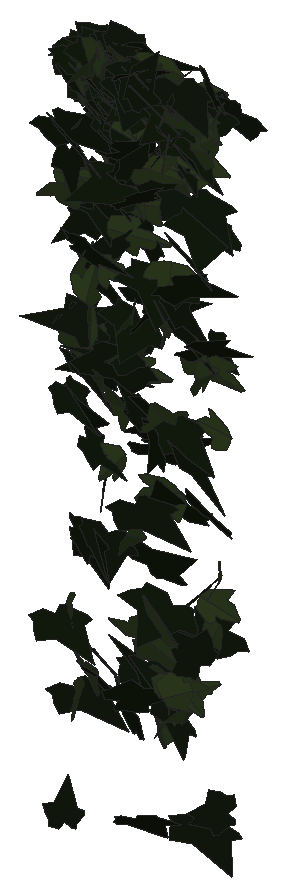
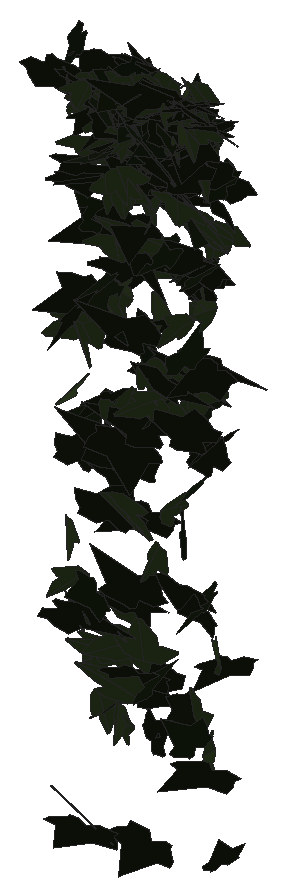
# SketchUp Ruby script. Lengths in millimetres.
U = 1.mm
M = Sketchup.active_model
def pt(a) = Geom::Point3d.new(a.map { |v| v * U })
def face(e, loops, mat)
  f = e.add_face(loops[0].map { |a| pt(a) })
  loops[1..].each { |l| e.add_face(l.map { |a| pt(a) }).erase! }
  f.material = f.back_material = mat if mat
  f
end
# faces: each face lists its corners as indices into pts; further lists are holes
def faces(e, pts, list, mat = nil) = list.each { |f| face(e, (f[0].is_a?(Array) ? f : [f]).map { |l| l.map { |i| pts[i] } }, mat) }
# xy, xz, yz: faces in a plane at the given z, y or x. An outline is a flat list of corners, or four numbers for a rectangle; further outlines are holes
def ring(l) = l.size == 4 ? [[l[0], l[1]], [l[2], l[1]], [l[2], l[3]], [l[0], l[3]]] : l.each_slice(2).to_a
def flat(e, list, mat, &to3) = list.each { |f| face(e, (f[0].is_a?(Array) ? f : [f]).map { |l| ring(l).map { |u, v| to3.(u, v) } }, mat) }
def xy(e, z, list, mat = nil) = flat(e, list, mat) { |x, y| [x, y, z] }
def xz(e, y, list, mat = nil) = flat(e, list, mat) { |x, z| [x, y, z] }
def yz(e, x, list, mat = nil) = flat(e, list, mat) { |y, z| [x, y, z] }
def lines(e, pts, list) = list.each { |a, b| e.add_line(pt(pts[a]), pt(pts[b])) }
# prism: a flat outline (further loops are holes) pulled along v
def prism(e, loops, v, mat = nil)
  f = face(e, loops, mat); d = Geom::Vector3d.new(v.map { |x| x * U })
  f.pushpull(f.normal.samedirection?(d) ? d.length : -d.length)
end
def box(e, o, s, mat = nil) = prism(e, [[o, [o[0] + s[0], o[1], o[2]], [o[0] + s[0], o[1] + s[1], o[2]], [o[0], o[1] + s[1], o[2]]]], [0, 0, s[2]], mat)
def at(x, y, z, deg = 0) = Geom::Transformation.translation(pt([x, y, z])) * Geom::Transformation.rotation(ORIGIN, Z_AXIS, deg.degrees)
def axes(o, x, y, z) = Geom::Transformation.new([*x, 0, *y, 0, *z, 0, *pt(o).to_a, 1])
def part(name) = M.definitions.add(name)
# library, detail: a bought-in or finely detailed component or shape, given as its bounding box
def library(name, o, s) = part(name).tap { |d| box(d.entities, o, s) }
def detail(e, o, s) = box(e.add_group.entities, o, s)
def put(e, d, t, mat = nil) = e.add_instance(d, t).tap { |i| i.material = mat if mat }
def group(e, t, mat = nil) = e.add_group.tap { |g| g.transformation = t; g.material = mat if mat }.entities
root = M.entities
M.materials.add("efeu1").color = [18, 25, 13]
M.materials.add("efeu2").color = [43, 57, 29]
c1 = part("ivyleaf_9")
p = [[39.1,54.8,31.7],[34.5,51.8,30.2],[-5.3,25.2,17.3],[-17.9,28.3,20.9],[-21.6,21.7,17],[-20.2,4.3,5.3],
  [-22.9,-0.3,2.5],[-17.1,-4,-0.6],[-2,-2.1,-1.2],[-0.7,-15.4,-10.1],[16.6,-22.3,-16.7],[21.1,-15.1,-12.5],
  [32.7,-10.7,-11],[46.1,-1.8,-6.6],[30.8,11.2,3.8]]
faces(c1.entities,p,[[0,1,2,3,4,5,6,7,8,9,10,11,12,13,14]],"efeu1")
c2 = part("ivyleaf_10")
p = [[0,12.8,-0.8],[-1.5,51.3,-10.9],[-4.9,51,-11.6],[-13.6,26.5,-7.3],[-13.2,15.9,-4.6],[-21.1,19.3,-7.2],
  [-29.5,16.3,-8.3],[-29.2,8.3,-6.2],[-19.7,-9.8,0.5],[-7.6,-13,4],[1,-12.2,5.8],[-0.4,51.1,-11.1],
  [-1.5,51.1,-10.9],[1,-12.4,5.9],[16.9,-12.4,3.5],[35.1,9.1,-5.1],[35,12.9,-6.1],[20.5,16.4,-4.9],
  [15.8,15,-3.8],[15.3,27.6,-7.1],[12.8,31.3,-7.8]]
faces(c2.entities,p,[[0,1,2,3,4,5,6,7,8,9,10],[11,12,0,13,14,15,16,17,18,19,20]],"efeu2")
put(root,c1,axes([3016.5,906.6,724.8],[0.03199,-0.66358,-0.6588],[-0.00347,0.65889,-0.66371],[1.77963,0.01322,0.01055]))
put(root,c1,axes([3235.8,920.3,1050.6],[0.77001,-0.91344,0.16816],[0.11583,-0.15696,-0.999],[1.76387,0.40906,-0.00781]))
put(root,c1,axes([3163.6,892,1496.8],[-0.15428,0.62413,0.77413],[-0.13659,0.771,-0.62913],[-1.88759,-0.1068,-0.01775]))
put(root,c1,axes([3119.7,925.8,1438],[-1.17393,-0.41882,0.51172],[-0.83195,-0.26683,-0.74529],[0.94432,-0.75573,-0.02045]))
put(root,c1,axes([3132.1,929.1,1585],[-0.45462,-0.7398,0.46488],[-0.03422,-0.47768,-0.76941],[1.66255,-0.21213,0.11129]))
put(root,c1,axes([3026,920.8,1459.1],[-0.74129,0.0016,-0.76927],[1.42556,-0.1957,-0.37966],[-0.33362,-0.83975,0.08701]))
put(root,c1,axes([3236.7,894.7,1333.6],[0.02355,0.26448,-0.88],[0.15228,0.87643,0.26454],[1.74218,-0.08018,-0.01122]))
put(root,c1,axes([3145.6,904.1,1598.4],[-1.12891,0.71334,0.38975],[0.45858,-0.30651,0.92768],[1.47753,0.64016,0.00987]))
put(root,c1,axes([3271.4,922.3,965.5],[1.1347,-0.65239,0.21976],[-0.27641,0.16498,0.88377],[-1.28069,-0.61363,0.00397]))
put(root,c2,axes([3021.4,927.9,733.6],[0.09927,-0.14231,-0.80456],[0.31208,-0.78798,0.15001],[-1.52338,-0.1707,-0.0217]))
put(root,c2,axes([3200,926.2,1527.2],[-0.00712,0.38664,-0.74683],[0.00939,-0.74681,-0.38666],[-1.60052,-0.0061,0.00105]))
put(root,c1,axes([3064.1,926,1574],[1.27825,-0.56394,-0.15563],[0.28866,-0.061,0.87557],[-1.07535,-0.68672,0.05003]))
put(root,c1,axes([3011.8,923.9,1489.2],[0.73758,-0.69043,0.3946],[0.33043,-0.35491,-0.79151],[1.47698,0.42419,-0.01998]))
put(root,c1,axes([3175.2,930.5,1048.2],[0.21099,-0.24209,-0.83674],[1.11722,-0.60241,0.25207],[-1.22479,-0.59121,0.08579]))
put(root,c1,axes([3136.7,900.5,635.8],[0.42934,0.04435,0.93346],[1.63406,0.3693,-0.22504],[-0.70222,0.88648,0.04705]))
put(root,c1,axes([3040.8,919.7,1317],[0.77704,-0.32089,0.63116],[0.90562,-0.41516,-0.51889],[0.99788,0.62665,-0.02057]))
put(root,c2,axes([3072.9,899,1260.7],[0.31768,0.55295,-0.67549],[0.18244,0.67195,0.57375],[1.65135,-0.18061,0.06656]))
put(root,c1,axes([3217.5,923,1554.7],[-0.80889,0.32031,-0.6481],[0.78398,-0.51052,-0.52245],[-1.13068,-0.58313,0.1014]))
put(root,c2,axes([3146.6,905.7,1250.1],[0.0201,-0.71991,-0.55145],[-0.0438,0.55109,-0.71989],[1.72535,0.02238,-0.01185]))
put(root,c2,axes([3065.2,924.6,1213.5],[0.01128,0.62166,-0.62218],[0.05319,-0.62201,-0.62123],[-1.67307,-0.01558,-0.02394]))
put(root,c1,axes([3223.8,929.5,1363.6],[0.26083,-0.60882,0.63453],[0.47113,-0.58951,-0.61909],[1.60594,0.27183,0.07857]))
put(root,c2,axes([3071.1,923.2,1107.6],[-1.08171,0.36184,0.57297],[0.83651,-0.37236,0.67114],[0.98166,0.71602,0.05947]))
put(root,c1,axes([3127.5,925,1160.2],[-0.02278,-0.04915,-0.96158],[-1.04023,-0.79135,0.04726],[-1.5086,0.5464,-0.01806]))
put(root,c1,axes([3140.7,932.1,1226.8],[-0.7383,-0.8102,0.2561],[-0.17966,-0.23869,-0.89811],[1.60715,-0.39888,0.01725]))
put(root,c1,axes([3028.2,908.9,404.5],[-0.60671,-0.39713,0.63358],[0.80336,0.47294,0.50883],[-1.17469,0.52856,0.02075]))
put(root,c1,axes([3167.3,925.1,1624.7],[-1.62137,-0.22979,-0.15515],[0.29372,0.02347,-0.88219],[0.43837,-0.86561,0.01726]))
put(root,c2,axes([3271.9,900.3,1197.8],[-0.09284,-0.21112,-0.88256],[0.39565,0.85773,-0.21667],[1.68115,-0.21352,0.00226]))
put(root,c1,axes([3147.5,899.8,1435.6],[0.79698,0.55323,0.53455],[0.59256,0.43467,-0.69376],[-1.33885,0.5217,0.01116]))
put(root,c2,axes([3026.5,914.1,1408.9],[-0.9948,-0.63536,-0.25479],[0.32696,0.18856,-0.82264],[1.26112,-0.55007,0.0123]))
put(root,c1,axes([3035.6,927.8,1127.1],[0.66585,-0.77664,0.20114],[0.21496,-0.16957,-0.85119],[1.51166,0.3662,0.03244]))
put(root,c2,axes([3207.5,912.1,756.8],[-1.03385,0.5754,-0.56238],[-0.75433,0.39914,0.79123],[1.33261,0.67234,0.01158]))
put(root,c2,axes([3065.5,913.8,1615.3],[-0.22834,-0.80416,-0.39552],[0.08826,0.39294,-0.81299],[1.70329,-0.12816,-0.01089]))
put(root,c1,axes([3150.3,932.7,1581.7],[0.31999,-0.57886,0.64341],[0.66315,-0.5547,-0.5901],[1.50779,0.36682,0.12299]))
put(root,c2,axes([3206.1,921.3,1334.5],[1.22811,0.5381,-0.09299],[-0.13681,-0.059,-0.84021],[-1.03024,0.64928,0.00072]))
put(root,c1,axes([3027.7,933.3,1048.1],[0.05351,-0.23036,0.88742],[0.72469,-0.80471,-0.22096],[1.58732,0.37516,0.07096]))
put(root,c1,axes([3066.6,926.1,1196.2],[-1.31861,0.12511,0.53559],[-1.01976,0.04091,-0.70268],[-0.23628,-0.87476,0.04374]))
put(root,c1,axes([3022.1,920.5,1082],[0.47438,-0.69712,-0.46598],[-0.30837,0.43693,-0.74033],[1.5658,0.29725,-0.00463]))
put(root,c2,axes([3211.4,921.6,682.1],[1.267,0.15294,0.54034],[0.97961,0.1689,-0.68197],[-0.42735,0.84061,0.03871]))
put(root,c2,axes([3219.8,909,671.3],[0.4764,0.20234,-0.90415],[1.31611,0.58252,0.32181],[1.17357,-0.73541,0.00614]))
put(root,c1,axes([3183.5,932.3,1309],[-1.2112,-0.66708,-0.29739],[0.39205,0.21449,-0.92196],[1.33361,-0.66891,0.00094]))
put(root,c2,axes([3034.2,924,1168.9],[-0.26087,-0.00409,-0.96092],[1.79905,-0.17506,-0.1341],[-0.32875,-0.95473,0.0287]))
put(root,c1,axes([3264.4,934.2,1420.5],[-1.06024,-0.68406,-0.15095],[0.19463,0.11137,-0.88216],[1.31895,-0.56632,0.00884]))
put(root,c2,axes([3121,913.8,1091.2],[0.69764,-0.22428,-0.77737],[-0.75589,0.69364,-0.38741],[1.34153,0.50747,0.18597]))
put(root,c1,axes([3208.9,933.6,1242.7],[0.79091,-0.76758,0.18436],[0.19312,-0.15468,-0.87272],[1.48995,0.42751,0.01525]))
put(root,c1,axes([3007.6,919.7,1504.4],[0.14455,-0.0471,-0.905],[1.13121,0.68814,0.01406],[1.30194,-0.59267,0.08826]))
put(root,c1,axes([3215.2,924,1086.1],[0.32906,-0.71736,-0.57502],[-0.18495,0.56756,-0.73727],[1.73995,0.196,0.03038]))
put(root,c1,axes([3086.7,935.3,1464.6],[-0.1513,-0.00027,0.88074],[0.91882,-0.73964,0.04335],[1.40196,0.48472,0.06664]))
put(root,c1,axes([3263.2,910.4,735.4],[-0.43663,0.59231,0.8468],[-0.6175,0.78226,-0.63507],[-1.86729,-0.39719,0.012]))
put(root,c1,axes([3215.3,928.6,1625.8],[-0.45933,-0.6222,-0.57073],[0.47956,0.51346,-0.66632],[1.53367,-0.3469,0.03741]))
put(root,c1,axes([3131.6,927.2,1177.7],[-1.51791,0.37027,0.39319],[-0.68532,0.15809,-0.87928],[-0.7661,-0.87505,0.00752]))
put(root,c1,axes([3151.1,926.6,1615.4],[1.34169,-0.49975,-0.12423],[-0.15909,0.09677,-0.8636],[0.96707,0.70926,0.03029]))
put(root,c2,axes([3050.7,934.9,628.1],[-1.03805,0.41996,0.55461],[0.84331,-0.33359,0.68835],[1.0207,0.70271,-0.00468]))
put(root,c1,axes([3127.2,914.3,1499.4],[1.12247,0.22043,0.72035],[1.26227,0.28189,-0.62928],[-0.67987,0.88729,0.02096]))
put(root,c2,axes([3158.4,919.7,1483.8],[-0.61294,-0.20641,-0.80724],[1.371,0.36593,-0.38097],[0.79688,-0.78832,0.03453]))
put(root,c1,axes([3205,927.3,1282.8],[0.90994,-0.6847,-0.38993],[-0.35624,0.34435,-0.83417],[1.4567,0.51192,0.03958]))
put(root,c2,axes([3023,945.8,591.7],[0.2596,-0.29183,0.87678],[0.80792,-0.76744,-0.32148],[1.56213,0.44541,0.02056]))
put(root,c1,axes([3205.2,943.4,1569.5],[-1.13814,-0.53068,0.26285],[-0.37501,-0.17398,-0.79953],[1.06289,-0.62964,-0.00062]))
put(root,c2,axes([3200.5,915,1251.7],[-0.17117,0.37181,-0.81824],[-0.568,0.76331,0.37965],[1.61345,0.30816,0.04685]))
put(root,c1,axes([3061.7,926.2,640.9],[1.49573,-0.2609,-0.21098],[-0.38053,0.06735,-0.82808],[0.51282,0.81094,0.0009]))
put(root,c1,axes([3250.1,916.2,1225.6],[1.06548,0.41629,0.59108],[0.91847,0.34146,-0.69757],[-1.02452,0.73905,-0.01065]))
put(root,c2,axes([3064.5,931.2,1627.5],[0.9873,-0.6228,-0.29877],[-0.37561,0.22443,-0.81051],[1.25984,0.55498,-0.00751]))
put(root,c1,axes([3187.5,931.6,1525.4],[-0.69255,0.6912,-0.30489],[0.27751,-0.26779,-0.78112],[-1.41075,-0.392,-0.00398]))
put(root,c1,axes([3142.9,929.8,1444.2],[-0.43917,-0.05903,0.8526],[1.59134,-0.19839,0.21256],[0.33667,0.86071,0.10747]))
put(root,c1,axes([3141.5,933.1,1077],[-0.23769,-0.72973,0.45929],[0.15503,0.45202,0.74033],[-1.63368,0.14907,0.00343]))
put(root,c1,axes([3189.4,947.2,613.8],[0.04591,-0.82645,0.28701],[0.05156,-0.28627,-0.82662],[1.66426,0.03167,0.01769]))
put(root,c1,axes([3185.7,944.3,783.6],[-1.56836,-0.48288,-0.08674],[0.13995,0.04608,-0.95511],[0.92317,-0.82733,-0.00257]))
put(root,c1,axes([3011.6,937.9,1573.3],[0.95627,-0.71675,-0.00209],[-0.00388,0.00112,-0.87532],[1.36411,0.50246,-0.00103]))
put(root,c2,axes([3011.1,934.6,1415.8],[0.26015,-0.19673,-0.77637],[1.4909,-0.1311,0.17114],[-0.31729,-0.77733,0.16762]))
put(root,c2,axes([3179.9,944.8,1071.6],[-0.80618,-0.63347,-0.44419],[-0.47773,-0.36649,0.76203],[-1.39283,0.49236,-0.00427]))
put(root,c1,axes([3181.4,946.8,1537.5],[0.55395,-0.77376,0.38072],[0.34464,-0.33802,-0.82542],[1.60464,0.33972,0.04585]))
put(root,c2,axes([3018.9,943.7,1573.3],[-0.79019,0.41173,-0.57655],[0.35845,-0.58007,-0.54987],[-1.29984,-0.41026,0.19885]))
put(root,c1,axes([3232,936.5,1449.2],[-0.55972,-0.5166,-0.75993],[0.94227,0.5831,-0.58799],[1.47329,-0.5692,0.08735]))
put(root,c2,axes([3225.2,931.8,1579],[-1.21506,-0.18733,-0.51249],[0.95175,0.11471,-0.6649],[0.41548,-0.8106,0.02435]))
put(root,c1,axes([3041.4,951.2,1353.8],[-0.05125,-0.00723,-0.85682],[0.44788,-0.82434,-0.00044],[-1.56805,-0.23522,0.02788]))
put(root,c2,axes([3042.8,919.1,1280.9],[0.31995,-0.30744,0.92992],[-0.61966,0.87232,0.34726],[-1.75802,-0.36342,0.04684]))
put(root,c2,axes([3122.1,949.8,1420.8],[-0.45389,0.26662,-0.79049],[0.49251,-0.75796,-0.33372],[-1.50942,-0.32749,0.12882]))
put(root,c2,axes([3182.1,936.2,1583.4],[0.68526,-0.77432,-0.22314],[-0.09085,0.22348,-0.85251],[1.53096,0.35985,0.04929]))
put(root,c2,axes([3255.5,953.6,1549],[-0.56066,0.2219,0.81755],[0.58302,-0.7791,0.32184],[1.50316,0.38495,0.18011]))
put(root,c1,axes([3139,932.5,930.1],[-0.16542,-0.34994,-0.84075],[0.67082,0.76582,-0.35519],[1.5981,-0.35768,0.06207]))
put(root,c2,axes([3170.5,936.2,716.6],[-1.50778,0.07311,-0.67145],[1.27343,-0.05628,-0.79559],[-0.17541,-1.03697,-0.00415]))
put(root,c1,axes([3129.9,926.5,1471.8],[-0.47597,0.51858,0.59693],[-0.51849,0.53123,-0.57564],[-1.41277,-0.36968,0.01015]))
put(root,c1,axes([3122.1,940.4,1606.2],[1.27898,-0.53776,0.07978],[0.11368,-0.05305,-0.86068],[1.0284,0.67466,-0.00408]))
put(root,c1,axes([3137.3,924.9,1619.8],[0.81769,0.74315,0.1304],[0.12793,0.11176,-0.8584],[-1.43026,0.43486,-0.00223]))
put(root,c1,axes([3050.4,934.4,1004.2],[0.85875,-0.53112,-0.52878],[-0.47761,0.47452,-0.69075],[1.34403,0.50797,0.09239]))
put(root,c1,axes([3217.1,941.5,1544.6],[-0.09698,-0.76734,-0.48789],[0.0211,0.48809,-0.76882],[1.73046,-0.04895,-0.01797]))
put(root,c2,axes([3185.1,952,1242.9],[0.58246,-0.68053,0.47277],[0.35148,-0.4353,-0.74613],[1.5374,0.35734,-0.00854]))
put(root,c1,axes([3106.4,939.8,1341.5],[-1.1618,0.56333,-0.07607],[0.10691,-0.05129,-0.83065],[-1.07656,-0.61303,-0.0004]))
put(root,c1,axes([3102.8,933.3,1578],[1.463,0.05488,-0.39208],[-0.75086,0.03492,-0.76862],[-0.06271,0.86221,0.05609]))
put(root,c1,axes([3055.5,953.4,1612.6],[-0.62933,-0.77131,0.05423],[-0.02561,-0.05323,-0.83916],[1.47135,-0.33083,0.00859]))
put(root,c1,axes([3129.6,935.5,576],[0.25378,-0.42054,0.73686],[-0.14931,0.7366,0.43459],[-1.6078,-0.13478,0.07595]))
put(root,c2,axes([3058.2,935.3,1601],[0.40126,-0.7276,-0.46431],[-0.00543,0.47738,-0.74936],[1.6427,0.17931,0.11094]))
put(root,c2,axes([3246.9,936.1,1532.1],[-0.60007,0.12301,0.8302],[-1.55694,0.15303,-0.33336],[-0.35675,-0.87477,0.05842]))
put(root,c1,axes([3258.2,935.3,1646.8],[0.99038,-0.38329,-0.62649],[-1.00202,0.34064,-0.64572],[0.97455,0.73976,-0.02726]))
put(root,c2,axes([3125.8,944.5,1166.8],[-0.42596,-0.92534,0.01728],[-0.00071,-0.01769,-0.95202],[1.76142,-0.22378,0.0038]))
put(root,c2,axes([3102.2,939.6,1626.1],[-1.31272,0.46227,-0.04073],[0.06058,-0.02565,-0.83032],[-0.88112,-0.69047,0.00358]))
put(root,c2,axes([3187.2,933.1,580.3],[0.71042,-0.29831,0.723],[-1.10589,0.43047,0.47761],[-0.99637,-0.69048,-0.0146]))
put(root,c2,axes([3249.5,939,1195.4],[-1.2336,-0.09948,-0.60288],[1.13359,0.09329,-0.65576],[0.25954,-0.88028,-0.00137]))
put(root,c1,axes([3094.9,947.7,1522.3],[-0.92806,-0.47094,-0.5863],[0.88455,0.36061,-0.67621],[1.12517,-0.67193,0.04801]))
put(root,c2,axes([3060.2,935,1421.9],[0.4104,-0.19118,-0.90246],[-1.32683,0.57316,-0.288],[1.14976,0.72967,-0.01023]))
put(root,c2,axes([3040.7,945.6,1514.4],[0.1265,-0.85038,-0.03459],[0.00369,0.03485,-0.85296],[1.61978,0.06633,0.00464]))
put(root,c1,axes([3099.8,961.4,1520.8],[-0.56583,-0.57673,0.50695],[-0.12178,-0.52312,-0.63265],[1.45631,-0.26783,0.14406]))
put(root,c1,axes([3148.1,945.6,676.5],[-0.48286,-0.54509,-0.63173],[0.61071,0.54577,-0.59979],[1.46589,-0.40693,0.04179]))
put(root,c2,axes([3135.9,948.2,717.8],[-1.62994,-0.13948,0.0913],[0.17289,0.01019,0.86769],[-0.26602,0.86121,0.00452]))
put(root,c2,axes([3278.6,935,862.5],[0.11288,-0.60517,-0.65708],[-0.13291,0.65337,-0.60806],[1.69493,0.09154,-0.00392]))
put(root,c1,axes([3141.7,952.8,651.9],[0.18676,-0.90153,0.2624],[-0.02483,0.26249,0.90673],[-1.78681,-0.09788,0.01482]))
put(root,c1,axes([3057.3,956.8,911.4],[0.07087,0.31494,0.82233],[-0.3632,-0.80062,0.31527],[1.63609,-0.19137,0.03437]))
put(root,c2,axes([3124.2,946.2,1526.9],[1.20968,0.67014,-0.01474],[-0.03719,-0.00178,-0.92353],[-1.27519,0.63577,0.01295]))
put(root,c2,axes([3209.1,948.1,619.9],[-0.25087,-0.91856,-0.06434],[0.02262,0.06329,-0.92796],[1.75233,-0.13232,0.00277]))
put(root,c1,axes([3117.9,945.4,1070.1],[0.64341,-0.16051,0.79315],[1.50112,-0.12685,-0.36186],[0.34438,0.85281,0.09545]))
put(root,c1,axes([3131,964,1562.1],[-1.301,-0.41977,0.28887],[-0.14222,-0.39553,-0.75161],[0.95932,-0.62793,0.28033]))
put(root,c2,axes([3077.2,965.2,970],[-0.33407,-0.17666,0.8406],[0.37561,-0.84331,-0.13602],[1.59104,0.16199,0.20861]))
put(root,c1,axes([3052.4,932.1,1418.5],[0.24669,0.51972,0.62303],[-0.0298,0.63241,-0.52429],[-1.54385,0.07084,0.10967]))
put(root,c2,axes([3095.8,949.3,1346.4],[0.16642,-0.13092,-0.85883],[1.63203,-0.12532,0.10641],[-0.26497,-0.85412,0.11603]))
put(root,c1,axes([3066.3,958.1,1504.1],[0.59109,-0.53856,0.66865],[1.00969,-0.43869,-0.59975],[1.28476,0.59254,0.16371]))
put(root,c2,axes([3266.2,959.1,1078.4],[-0.65182,0.61,0.50448],[-0.00949,-0.55133,0.66326],[1.50652,0.26045,0.22245]))
put(root,c2,axes([3074.4,933.4,1611.8],[0.26925,-0.15741,-0.87203],[0.0835,0.88323,-0.15232],[1.6844,-0.01862,0.14694]))
put(root,c1,axes([3021.3,933.2,1195.7],[0.04195,0.08481,-0.91651],[-0.31339,0.90235,0.07954],[1.7235,0.16201,0.03677]))
put(root,c1,axes([3066.5,956.4,850.3],[-1.22177,-0.22742,-0.54099],[0.98604,0.15695,-0.68077],[0.52457,-0.82471,0.01962]))
put(root,c2,axes([3140.4,957.8,1517.4],[0.84519,-0.66404,0.31124],[0.4531,-0.21361,-0.79544],[1.32013,0.49845,0.07375]))
put(root,c1,axes([3028.7,958.9,831.2],[-0.52622,-0.04987,-0.81742],[1.5578,-0.04446,-0.27415],[-0.04993,-0.86177,0.06145]))
put(root,c1,axes([3012.2,953.3,1596.8],[0.0726,-0.75855,-0.42726],[0.15784,0.42889,-0.75404],[1.64939,-0.00765,0.09097]))
put(root,c1,axes([3136.5,933.7,1206.5],[0.27024,0.11651,0.91878],[0.88495,0.7949,-0.17266],[-1.52437,0.48212,0.06264]))
put(root,c2,axes([3117.8,939.5,876.4],[-0.1213,-0.52352,-0.73971],[0.29911,0.72391,-0.52588],[1.69859,-0.16486,0.03978]))
put(root,c1,axes([3020,944.7,846.7],[1.03775,-0.43197,-0.62968],[-0.81135,0.46972,-0.6914],[1.20572,0.68788,0.0767]))
put(root,c1,axes([3188.5,965.3,1502.8],[0.0903,-0.84082,0.1988],[0.10601,-0.19571,-0.84104],[1.64094,0.05891,0.0434]))
put(root,c2,axes([3250.6,945.3,1185.9],[0.5766,-0.60334,-0.57966],[-0.38396,0.54562,-0.67335],[1.54537,0.36068,0.04898]))
put(root,c2,axes([3148.9,965.4,1611],[0.37723,-0.60512,0.54647],[0.44574,-0.49643,-0.63466],[1.48638,0.30244,0.05163]))
put(root,c2,axes([3163.7,950.8,647.8],[-0.66458,-0.15127,0.8439],[1.51356,0.28326,0.37984],[-0.60958,0.86825,0.0231]))
put(root,c2,axes([3226.3,955.5,1498.9],[1.21596,0.52676,-0.11076],[-0.146,-0.08105,-0.82794],[-1.014,0.64335,-0.01361]))
put(root,c2,axes([3236.8,951,1577.7],[1.40887,-0.37579,-0.26062],[-0.24737,0.30254,-0.80542],[0.83447,0.72414,0.20125]))
put(root,c2,axes([3140.5,949.8,1614.5],[-0.46532,-0.75401,-0.33591],[0.32866,0.29586,-0.7898],[1.53623,-0.29168,0.06722]))
put(root,c1,axes([3105.3,947.3,1615.5],[1.44869,0.06902,-0.43395],[-0.82854,0.00065,-0.76352],[-0.1135,0.87619,0.03475]))
put(root,c1,axes([3102.8,961.6,1522],[-0.16574,-0.79484,-0.19801],[0.0887,0.194,-0.79922],[1.55644,-0.09569,0.02446]))
put(root,c2,axes([3180.7,944.1,605.6],[-0.02811,-0.60436,-0.67066],[0.01484,0.67064,-0.60452],[1.71814,-0.01568,-0.00575]))
put(root,c2,axes([3252,959.5,761.4],[1.07792,-0.63545,0.04914],[0.06235,-0.03662,-0.85122],[1.21139,0.56732,0.00009]))
put(root,c1,axes([3055.5,969.7,1584.8],[-0.74503,-0.6806,0.22902],[-0.23399,-0.19347,-0.78509],[1.34651,-0.4102,-0.00971]))
put(root,c1,axes([3029.7,963.4,1552.1],[0.08348,-0.85651,-0.16835],[-0.04079,0.16746,-0.85754],[1.6608,0.04716,-0.0126]))
put(root,c1,axes([3032.6,966.4,1367.1],[0.1457,-0.80206,0.06377],[0.05416,-0.06132,-0.8054],[1.53034,0.07853,0.02243]))
put(root,c1,axes([3145,961.9,1003.3],[1.55652,0.26641,0.14666],[-0.265,-0.04607,0.86014],[0.51455,-0.82961,-0.00066]))
put(root,c1,axes([3265,962.2,1590],[-1.53198,0.15235,0.20223],[-0.37263,0.05283,-0.8191],[-0.30555,-0.82828,-0.01504]))
put(root,c1,axes([3214,950.5,1540.1],[-0.80281,0.57027,0.48504],[-0.64844,0.34951,-0.70722],[-1.26872,-0.53948,0.05454]))
put(root,c1,axes([3027,961.4,1098.5],[0.51355,-0.16319,0.8108],[1.35638,-0.38687,-0.31505],[0.79868,0.76193,0.01369]))
put(root,c1,axes([3181.6,965.5,922.6],[1.32379,-0.20347,0.51118],[-0.93602,0.1394,0.7247],[-0.46936,-0.85186,-0.00351]))
put(root,c2,axes([3171,956.8,1446.3],[-1.29483,-0.43358,-0.179],[0.2875,0.09603,-0.80676],[0.84518,-0.69691,0.0002]))
put(root,c2,axes([3142.8,962.1,1626.4],[1.11142,0.57092,-0.23145],[-0.39416,-0.11842,-0.81464],[-1.10423,0.61691,0.05783]))
put(root,c2,axes([3071.8,965.7,1607.9],[-0.22813,-0.82428,0.1953],[-0.1094,-0.18887,-0.83245],[1.60849,-0.12975,-0.02892]))
put(root,c1,axes([3124.5,948.6,421.4],[1.19635,0.53932,0.06963],[0.08276,0.05624,-0.82813],[-1.03163,0.62994,0.01432]))
put(root,c1,axes([3251.5,952.8,1218.6],[0.47639,-0.40223,-0.72318],[-0.71729,0.61722,-0.47374],[1.4021,0.45242,0.00335]))
put(root,c1,axes([3115,956.7,1158.9],[-0.66356,0.2625,0.75661],[-1.15385,0.45266,-0.43642],[-0.99589,-0.69937,0.00152]))
put(root,c1,axes([3295.5,961.7,1598.3],[0.2114,0.16435,-0.82452],[-1.35362,-0.42512,-0.18055],[-0.85324,0.71515,0.08215]))
put(root,c1,axes([3165,956.2,1028.8],[1.18739,0.67196,-0.27281],[0.35469,0.19924,0.91694],[1.33391,-0.65113,-0.00097]))
put(root,c2,axes([3167,962.2,1610.2],[-1.3794,0.22806,-0.39044],[0.69959,-0.13238,-0.75968],[-0.50114,-0.81254,0.01418]))
put(root,c1,axes([3051.2,973.6,1620],[-0.41606,-0.807,-0.0371],[0.18911,0.01128,-0.83091],[1.52582,-0.22145,0.09287]))
put(root,c1,axes([3151.5,975.7,1599.4],[0.40485,-0.79979,-0.11355],[0.03903,-0.11204,0.82755],[-1.53693,-0.21352,-0.0089]))
put(root,c2,axes([3259.4,962.5,1596.8],[0.47654,-0.78305,-0.18659],[0.00201,0.19573,-0.81998],[1.53202,0.24331,0.05911]))
put(root,c2,axes([3119,952.3,1574],[0.64341,0.57935,0.48627],[-0.02306,0.53671,-0.63102],[-1.43935,0.25038,0.22748]))
put(root,c1,axes([3101.1,966.5,1628.4],[-1.1738,0.23153,0.49701],[-0.9739,0.02557,-0.64691],[-0.37474,-0.79167,0.12446]))
put(root,c1,axes([3180.6,956.3,1548.3],[0.44645,-0.46284,-0.67913],[-0.44921,0.63856,-0.51672],[1.49826,0.32938,0.04744]))
put(root,c2,axes([3114.7,964.1,1601.2],[0.91923,0.66852,-0.04524],[-0.10409,-0.01624,-0.82401],[-1.27099,0.48483,0.03477]))
put(root,c1,axes([3023.8,961.7,1382],[-0.23419,-0.06856,-0.87052],[1.30036,0.53988,-0.1391],[1.0349,-0.69388,-0.02221]))
put(root,c2,axes([3171.1,962.3,949.6],[1.22216,-0.32282,-0.60773],[-1.02049,0.28627,-0.71864],[0.82088,0.83651,0.01141]))
put(root,c2,axes([3159.4,967.5,1472.1],[-0.63191,-0.78691,0.08326],[-0.05785,-0.07755,-0.85409],[1.5049,-0.3334,0.00213]))
put(root,c2,axes([3054.3,970.3,1567.1],[0.08169,-0.81362,0.15034],[0.00273,-0.15047,-0.81472],[1.57468,0.04247,-0.00639]))
put(root,c1,axes([3118.9,958.6,1548.2],[0.43231,-0.47507,-0.6384],[-0.10395,0.65303,-0.50539],[1.51094,0.18085,0.14789]))
put(root,c1,axes([3141.4,957.4,1351.7],[0.15317,-0.02272,-0.87671],[-1.65995,0.09002,-0.0824],[0.17459,0.87578,-0.01427]))
put(root,c2,axes([3103,965.9,1595.9],[0.92088,0.66196,-0.08873],[-0.14722,-0.05329,-0.81936],[-1.26255,0.48903,0.03082]))
put(root,c2,axes([3104.5,960.7,1439.6],[-0.62137,0.79351,0.09053],[-0.07942,0.08072,-0.85801],[-1.51793,-0.32905,0.00783]))
put(root,c1,axes([3050.7,971,1618.9],[-1.51184,0.24896,0.09282],[-0.2223,-0.06438,-0.82694],[-0.4542,-0.79718,0.09577]))
put(root,c1,axes([3127.5,972.3,818.1],[-0.35765,-0.10209,0.90296],[1.35667,-0.58843,0.08182],[1.07261,0.71022,0.19759]))
put(root,c2,axes([3170.8,961.6,1452.6],[-1.37426,0.23643,0.34734],[-0.61531,0.12846,-0.75955],[-0.51075,-0.79091,-0.01954]))
put(root,c1,axes([3008.8,977.8,1370],[0.33513,-0.79948,0.16462],[0.04679,-0.16314,-0.81857],[1.55279,0.17746,-0.01087]))
put(root,c1,axes([3034.8,961.9,1562.8],[0.68824,-0.55029,-0.57723],[-0.18541,0.59857,-0.63166],[1.50643,0.32508,0.18597]))
put(root,c2,axes([3084.5,972.1,1600.8],[0.99841,0.6027,-0.26902],[-0.34072,-0.20082,-0.79902],[-1.20905,0.55429,0.00302]))
put(root,c1,axes([3257.2,977.9,754.2],[-0.32358,-0.2,-0.85981],[-0.97385,-0.69118,0.26195],[-1.36904,0.53893,0.01688]))
put(root,c1,axes([3179.2,970.9,1502],[0.5952,-0.76868,-0.21066],[0.2688,0.27616,-0.79802],[1.49289,0.25674,0.22768]))
put(root,c2,axes([3110.8,956.7,1125.6],[-0.46013,-0.28773,-0.79689],[1.03019,0.58507,-0.37547],[1.24049,-0.59261,0.01623]))
put(root,c1,axes([3156.7,960.3,1049.8],[0.81936,0.78696,-0.27204],[-0.26348,-0.23433,-0.89698],[-1.56264,0.45215,0.0086]))
put(root,c1,axes([3069,964.8,1387.3],[1.17799,-0.39521,-0.35068],[-0.45915,0.26914,-0.72913],[0.89464,0.65852,0.08754]))
put(root,c1,axes([3062.6,977.4,1622.3],[0.15473,-0.82454,-0.07831],[-0.00345,0.07851,-0.82852],[1.57632,0.08111,0.00587]))
put(root,c1,axes([3025.9,979.6,1599.6],[-1.01837,-0.61574,-0.12557],[0.18124,0.08357,-0.81557],[1.18218,-0.54323,0.01686]))
put(root,c1,axes([3115.7,981.2,1584.3],[-0.34119,-0.80186,0.04268],[-0.01988,-0.0414,-0.82165],[1.52813,-0.17957,-0.00116]))
put(root,c1,axes([3006.2,964,580.5],[-0.10594,-0.38101,-0.81682],[0.50708,0.77484,-0.37959],[1.63871,-0.2644,0.06465]))
put(root,c2,axes([3245.8,958.5,804.7],[0.28082,0.56416,0.62273],[0.26053,0.60767,-0.58295],[-1.57785,0.20074,0.01458]))
put(root,c1,axes([3175.5,953.5,1600.4],[0.40606,0.53469,0.60036],[0.36871,0.56864,-0.57529],[-1.48497,0.2874,0.02132]))
put(root,c1,axes([3143.1,954,1568.2],[0.43934,0.59351,0.53115],[0.27986,0.51174,-0.63574],[-1.48979,0.27116,0.03721]))
put(root,c1,axes([3028.5,989.6,1229.6],[1.04116,-0.68574,-0.42646],[0.50173,-0.33523,0.87721],[-1.45269,-0.60726,-0.00268]))
put(root,c2,axes([3112.2,968.1,1388.4],[0.38833,0.04589,-0.87023],[1.65311,0.06139,0.2069],[0.1338,-0.89172,-0.03054]))
put(root,c2,axes([3131.9,977.6,1545],[0.31072,0.76137,-0.29058],[-0.09939,-0.28597,-0.77864],[-1.54781,0.17121,-0.00833]))
put(root,c1,axes([3186.3,973.9,1579.1],[-0.94443,0.65289,-0.17433],[-0.00203,-0.21704,-0.80981],[-1.28611,-0.4791,0.12929]))
put(root,c2,axes([3024.4,976.5,1597.2],[1.44991,0.29375,-0.05461],[-0.08236,-0.03951,-0.81622],[-0.56265,0.76276,-0.02125]))
put(root,c2,axes([3055,960,1271.2],[0.11633,0.52183,0.68495],[0.00094,0.68665,-0.52317],[-1.63882,0.03744,0.04832]))
put(root,c2,axes([3048.3,984.9,1544.4],[0.20337,-0.09981,0.80268],[1.29843,-0.42383,-0.14352],[0.82699,0.68999,0.02795]))
put(root,c1,axes([3163.3,975.2,1567.1],[0.05602,0.63866,-0.53812],[-0.22176,-0.53005,-0.63545],[-1.5739,0.09741,0.07038]))
put(root,c1,axes([3060.4,983.9,1569.8],[0.63993,0.21352,0.71521],[-1.13293,-0.39652,0.39823],[0.85698,-0.68363,-0.0076]))
put(root,c1,axes([3073.4,980.8,1586.4],[-0.91637,0.44735,-0.49059],[0.54565,-0.4065,-0.65207],[-1.1397,-0.55431,0.08227]))
put(root,c1,axes([3082.4,959.3,1543],[0.86956,0.44228,0.51735],[0.54865,0.43871,-0.62964],[-1.17345,0.53286,0.08898]))
put(root,c1,axes([3140.9,969.4,1413.6],[1.23986,0.26325,-0.48071],[-0.85422,-0.17226,-0.7026],[-0.5986,0.79108,0.00697]))
put(root,c2,axes([3175.7,975.2,1572.8],[0.58603,-0.75855,-0.17561],[0.00357,0.18957,-0.81555],[1.48186,0.29953,0.07142]))
put(root,c2,axes([3137.4,976.9,1551.9],[-1.27592,-0.48248,-0.10161],[0.3414,-0.07893,-0.8088],[0.8741,-0.67346,0.16758]))
put(root,c2,axes([3215.2,972.3,1599],[0.58315,0.77243,0.13693],[0.04253,0.13835,-0.83045],[-1.49241,0.30577,0.02984]))
put(root,c1,axes([3057.8,977.7,1494.8],[-1.35284,0.40271,-0.09212],[0.16051,-0.03801,-0.81693],[-0.76967,-0.71576,-0.00845]))
put(root,c1,axes([3121.5,974.8,1227.4],[0.03973,-0.0106,0.88885],[1.61331,-0.26741,-0.0231],[0.50929,0.84793,0.00382]))
put(root,c2,axes([3046.3,980.3,1471.5],[1.49851,-0.09526,0.19053],[0.35521,-0.04317,-0.79286],[0.19542,0.80894,-0.01987]))
put(root,c1,axes([3212,960.8,791.7],[-0.43169,0.62464,-0.5285],[-0.46275,0.47221,0.66245],[1.4869,0.32831,0.05273]))
put(root,c1,axes([3012.1,991.8,632.6],[0.3781,-0.5933,0.60102],[0.511,-0.54102,-0.62282],[1.52391,0.32862,0.05972]))
put(root,c1,axes([3035.2,970.2,1573.3],[1.20987,0.37801,-0.34333],[-0.68457,-0.05768,-0.72951],[-0.68986,0.72019,0.12178]))
put(root,c1,axes([3095,977,1609.6],[0.59127,-0.0639,0.77088],[1.44619,-0.13014,-0.31702],[0.2753,0.82087,0.00975]))
put(root,c1,axes([3212.9,981.7,428.7],[-0.67612,-0.45486,-0.67218],[0.80481,0.52255,-0.5771],[1.31844,-0.55224,0.00757]))
put(root,c1,axes([3026.1,971.8,1515.5],[0.42164,-0.01211,0.8427],[1.57292,0.17379,-0.21478],[-0.31417,0.85383,0.05566]))
put(root,c2,axes([3032.7,982.2,1596.7],[-0.11974,-0.81765,-0.05684],[-0.02955,0.05818,-0.81982],[1.55962,-0.06167,-0.0199]))
put(root,c2,axes([3130.9,977.8,1546.7],[0.22675,0.81646,0.10287],[0.00819,0.10332,-0.82504],[-1.56614,0.11875,0.01058]))
put(root,c1,axes([3255.8,980.2,462.6],[-1.3225,0.55146,0.08852],[-0.14028,0.04951,-0.88709],[-1.05368,-0.69874,0.007]))
put(root,c1,axes([3130,970.6,1552.8],[-0.71953,0.79541,0.46608],[-0.35183,0.42811,-0.88056],[-1.71893,-0.42058,-0.01487]))
